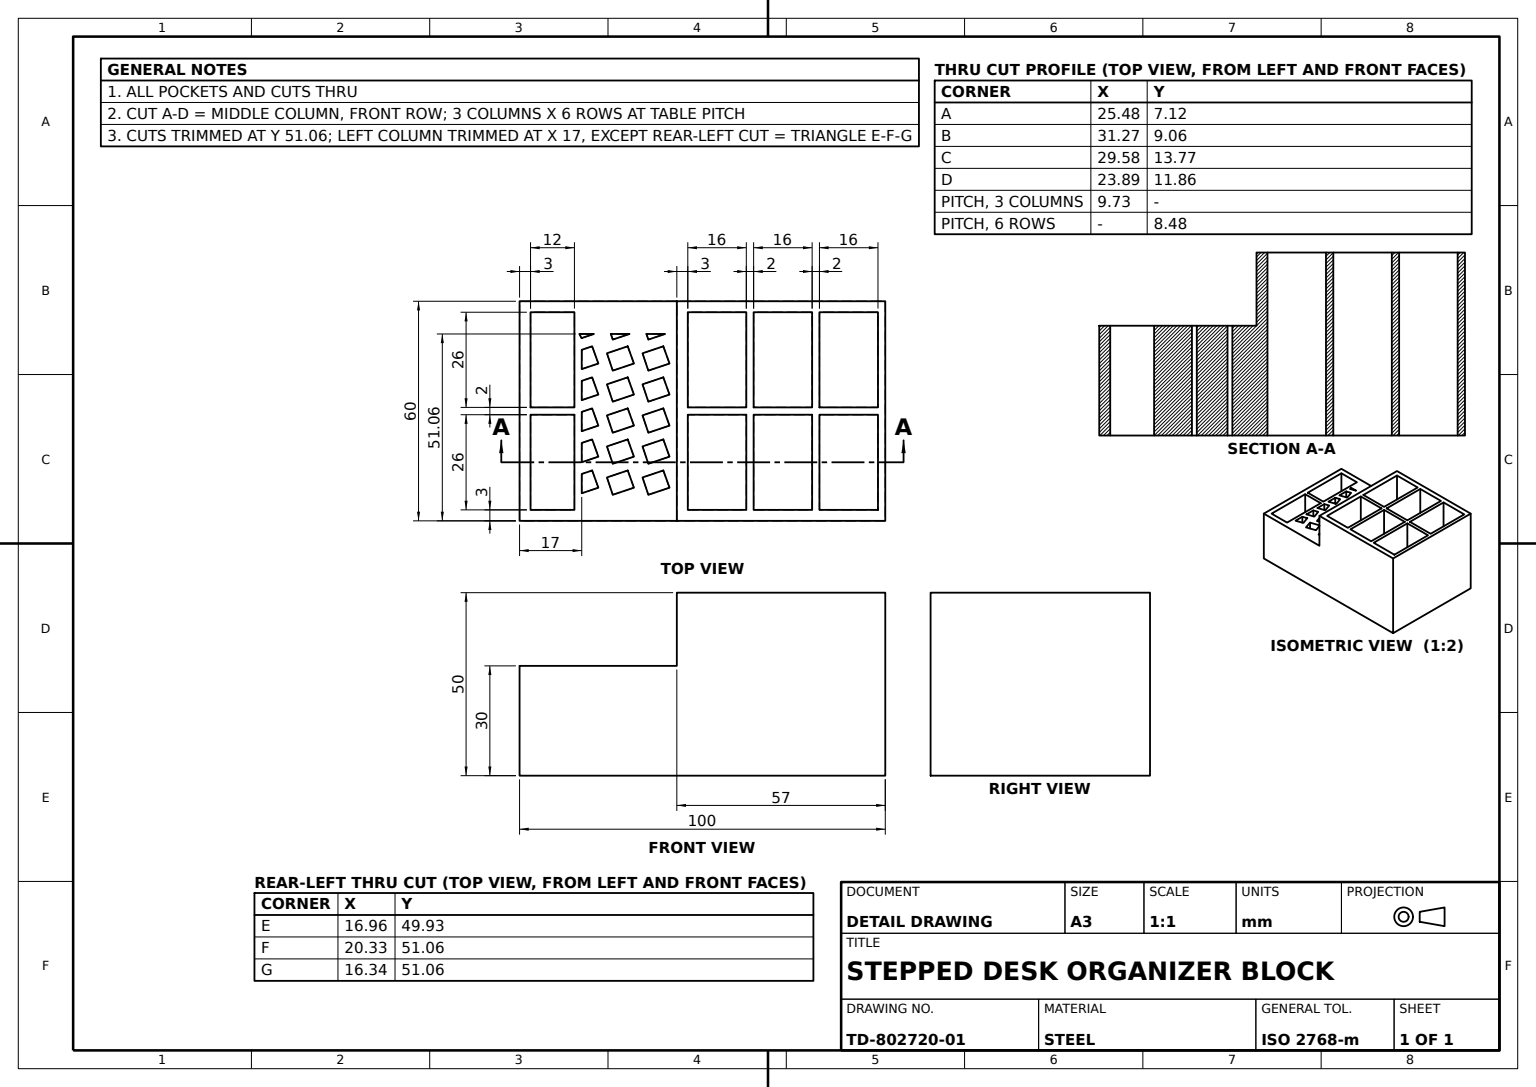
solid
v1 (12,5.599473,-1)
v2 (12,5.599473,-27)
e1 v1 v2 LINE
v3 (12,55.599473,-1)
e2 v1 v3 LINE
v4 (12,55.599473,-27)
e3 v3 v4 LINE
e4 v2 v4 LINE
face PLANE(AX(P(12,5.599473,-1),D(1,0,0),D(0,1,0))) rev [-e1 e2 e3 -e4]
v5 (30,5.599473,-27)
v6 (14,5.599473,-27)
e5 v5 v6 LINE
v7 (30,55.599473,-27)
e6 v5 v7 LINE
v8 (14,55.599473,-27)
e7 v7 v8 LINE
e8 v6 v8 LINE
face PLANE(AX(P(14,5.599473,-27),D(0,0,-1),D(-1,0,0))) rev [-e5 e6 e7 -e8]
v9 (-30.149435,35.599473,-0.727667)
v10 (-33,35.599473,0.227423)
e9 v9 v10 LINE
v11 (-33,5.599473,0.227423)
e10 v11 v10 LINE
v12 (-30.149435,5.599473,-0.727667)
e11 v11 v12 LINE
e12 v12 v9 LINE
face PLANE(AX(P(-33,-4.332499,0.227423),D(-0.317694802,0,-0.948193025),D(-0.948193025,0,0.317694802))) rev [e9 -e10 e11 e12]
v13 (-28.457896,5.599473,3.977511)
e13 v12 v13 LINE
v14 (-28.457896,35.599473,3.977511)
e14 v13 v14 LINE
e15 v14 v9 LINE
face PLANE(AX(P(-30.149435,-4.332499,-0.727667),D(0.941035568,0,-0.338307639),D(-0.338307639,0,-0.941035568))) rev [e13 e14 e15 -e12]
v15 (-4,55.599473,-27)
v16 (-4,55.599473,-1)
e16 v15 v16 LINE
v17 (-4,5.599473,-1)
e17 v17 v16 LINE
v18 (-4,5.599473,-27)
e18 v18 v17 LINE
e19 v18 v15 LINE
face PLANE(AX(P(-4,5.599473,-1),D(-1,0,0),D(0,-1,0))) rev [e16 -e17 -e18 e19]
e20 v4 v15 LINE
e21 v2 v18 LINE
face PLANE(AX(P(-4,5.599473,-27),D(0,0,-1),D(-1,0,0))) rev [e4 e20 -e19 -e21]
v19 (30,5.599473,1)
v20 (30,55.599473,1)
e22 v19 v20 LINE
v21 (14,55.599473,1)
e23 v20 v21 LINE
v22 (14,5.599473,1)
e24 v22 v21 LINE
e25 v19 v22 LINE
face PLANE(AX(P(14,5.599473,1),D(0,0,-1),D(-1,0,0))) rev [e22 e23 -e24 -e25]
v23 (14,55.599473,27)
v24 (30,55.599473,27)
e26 v23 v24 LINE
e27 v21 v23 LINE
e28 v24 v20 LINE
v25 (30,55.599473,-1)
e29 v25 v7 LINE
v26 (14,55.599473,-1)
e30 v26 v25 LINE
e31 v8 v26 LINE
v27 (12,55.599473,27)
v28 (12,55.599473,1)
e32 v27 v28 LINE
v29 (-4,55.599473,27)
e33 v29 v27 LINE
v30 (-4,55.599473,1)
e34 v30 v29 LINE
e35 v28 v30 LINE
v31 (32,55.599473,-1)
v32 (48,55.599473,-1)
e36 v31 v32 LINE
v33 (32,55.599473,-27)
e37 v33 v31 LINE
v34 (48,55.599473,-27)
e38 v34 v33 LINE
e39 v32 v34 LINE
e40 v16 v3 LINE
v35 (48,55.599473,27)
v36 (48,55.599473,1)
e41 v35 v36 LINE
v37 (32,55.599473,27)
e42 v37 v35 LINE
v38 (32,55.599473,1)
e43 v38 v37 LINE
e44 v36 v38 LINE
v39 (50,55.599473,30)
v40 (50,55.599473,-30)
e45 v39 v40 LINE
v41 (-7,55.599473,-30)
e46 v40 v41 LINE
v42 (-7,55.599473,30)
e47 v42 v41 LINE
e48 v39 v42 LINE
face PLANE(AX(P(50,55.599473,30),D(0,-1,0),D(1,0,0))) rev [-e26 -e27 -e23 -e28] [-e29 -e30 -e31 -e7] [-e32 -e33 -e34 -e35] [-e36 -e37 -e38 -e39] [-e20 -e3 -e40 -e16] [-e41 -e42 -e43 -e44] [e45 e46 -e47 -e48]
v43 (-10.691538,35.599473,16.234119)
v44 (-16.380696,35.599473,18.140288)
e49 v43 v44 LINE
v45 (-16.380696,5.599473,18.140288)
e50 v45 v44 LINE
v46 (-10.691538,5.599473,16.234119)
e51 v45 v46 LINE
e52 v46 v43 LINE
face PLANE(AX(P(-16.380696,-4.332499,18.140288),D(-0.317694802,0,-0.948193025),D(-0.948193025,0,0.317694802))) rev [e49 -e50 e51 e52]
v47 (-9,5.599473,-12.984275)
v48 (-9,35.599473,-12.984275)
e53 v47 v48 LINE
v49 (-10.691538,35.599473,-17.689453)
e54 v48 v49 LINE
v50 (-10.691538,5.599473,-17.689453)
e55 v50 v49 LINE
e56 v50 v47 LINE
face PLANE(AX(P(-10.691538,-4.332499,-17.689453),D(0.941035568,0,-0.338307639),D(-0.338307639,0,-0.941035568))) rev [e53 e54 -e55 e56]
v51 (-33,35.599473,-8.25347)
v52 (-33,35.599473,-2.981537)
e57 v51 v52 LINE
v53 (-33,5.599473,-2.981537)
e58 v53 v52 LINE
v54 (-33,5.599473,-8.25347)
e59 v53 v54 LINE
e60 v54 v51 LINE
face PLANE(AX(P(-33,-4.332499,-8.25347),D(-1,0,0),D(0,-1,0))) rev [e57 -e58 e59 e60]
v55 (-24.521549,35.599473,5.918339)
v56 (-18.728948,35.599473,3.977511)
e61 v55 v56 LINE
v57 (-18.728948,5.599473,3.977511)
e62 v57 v56 LINE
v58 (-24.521549,5.599473,5.918339)
e63 v57 v58 LINE
e64 v58 v55 LINE
face PLANE(AX(P(-18.728948,-4.332499,3.977511),D(0.317694802,0,0.948193025),D(0.948193025,0,-0.317694802))) rev [e61 -e62 e63 e64]
v59 (-33.041679,5.599473,-19.929358)
v60 (-33.663374,5.599473,-21.060067)
e65 v59 v60 LINE
v61 (-33.663374,35.599473,-21.060067)
e66 v60 v61 LINE
v62 (-33.041679,35.599473,-19.929358)
e67 v61 v62 LINE
e68 v59 v62 LINE
face PLANE(AX(P(-33.041679,-4.332499,-19.929358),D(-0.87627987,0,0.481802437),D(0.481802437,0,0.87627987))) rev [e65 e66 e67 -e68]
v63 (-10.691538,35.599473,7.753226)
v64 (-16.380696,35.599473,9.659395)
e69 v63 v64 LINE
v65 (-16.380696,5.599473,9.659395)
e70 v65 v64 LINE
v66 (-10.691538,5.599473,7.753226)
e71 v65 v66 LINE
e72 v66 v63 LINE
face PLANE(AX(P(-16.380696,-4.332499,9.659395),D(-0.317694802,0,-0.948193025),D(-0.948193025,0,0.317694802))) rev [e69 -e70 e71 e72]
v67 (32,5.599473,27)
e73 v67 v37 LINE
v68 (32,5.599473,1)
e74 v68 v67 LINE
e75 v68 v38 LINE
face PLANE(AX(P(32,5.599473,1),D(-1,0,0),D(0,-1,0))) rev [-e73 -e74 e75 e43]
v69 (-28.457896,35.599473,-12.984275)
v70 (-30.149435,35.599473,-17.689453)
e76 v69 v70 LINE
v71 (-30.149435,5.599473,-17.689453)
e77 v71 v70 LINE
v72 (-28.457896,5.599473,-12.984275)
e78 v71 v72 LINE
e79 v72 v69 LINE
face PLANE(AX(P(-30.149435,-4.332499,-17.689453),D(0.941035568,0,-0.338307639),D(-0.338307639,0,-0.941035568))) rev [e76 -e77 e78 e79]
v73 (-9,5.599473,3.977511)
v74 (-14.7926,5.599473,5.918339)
e80 v73 v74 LINE
v75 (-14.7926,35.599473,5.918339)
e81 v74 v75 LINE
v76 (-9,35.599473,3.977511)
e82 v75 v76 LINE
e83 v73 v76 LINE
face PLANE(AX(P(-9,-4.332499,3.977511),D(0.317694802,0,0.948193025),D(0.948193025,0,-0.317694802))) rev [e80 e81 e82 -e83]
v77 (-4,5.599473,1)
e84 v77 v30 LINE
v78 (-4,5.599473,27)
e85 v78 v29 LINE
e86 v77 v78 LINE
face PLANE(AX(P(-4,5.599473,1),D(-1,0,0),D(0,-1,0))) rev [e84 e34 -e85 -e86]
e87 v17 v1 LINE
face PLANE(AX(P(-4,5.599473,-1),D(0,0,1),D(1,0,0))) rev [-e2 -e87 e17 e40]
v79 (-24.521549,35.599473,-11.043447)
v80 (-18.728948,35.599473,-12.984275)
e88 v79 v80 LINE
v81 (-18.728948,5.599473,-12.984275)
e89 v81 v80 LINE
v82 (-24.521549,5.599473,-11.043447)
e90 v81 v82 LINE
e91 v82 v79 LINE
face PLANE(AX(P(-18.728948,-4.332499,-12.984275),D(0.317694802,0,0.948193025),D(0.948193025,0,-0.317694802))) rev [e88 -e89 e90 e91]
v83 (-20.420486,5.599473,-9.20856)
v84 (-20.420486,35.599473,-9.20856)
e92 v83 v84 LINE
v85 (-26.109645,35.599473,-7.302391)
e93 v84 v85 LINE
v86 (-26.109645,5.599473,-7.302391)
e94 v86 v85 LINE
e95 v86 v83 LINE
face PLANE(AX(P(-26.109645,-4.332499,-7.302391),D(-0.317694802,0,-0.948193025),D(-0.948193025,0,0.317694802))) rev [e92 e93 -e94 e95]
v87 (48,5.599473,1)
e96 v87 v36 LINE
v88 (48,5.599473,27)
e97 v88 v87 LINE
e98 v88 v35 LINE
face PLANE(AX(P(48,5.599473,1),D(1,0,0),D(0,1,0))) rev [e41 -e96 -e97 e98]
v89 (-33,5.599473,17.189209)
v90 (-33,35.599473,17.189209)
e99 v89 v90 LINE
v91 (-30.149435,5.599473,16.234119)
e100 v89 v91 LINE
v92 (-30.149435,35.599473,16.234119)
e101 v91 v92 LINE
e102 v92 v90 LINE
face PLANE(AX(P(-33,-4.332499,17.189209),D(-0.317694802,0,-0.948193025),D(-0.948193025,0,0.317694802))) rev [-e99 e100 e101 e102]
v93 (-14.7926,35.599473,-2.562554)
v94 (-9,35.599473,-4.503382)
e103 v93 v94 LINE
v95 (-9,5.599473,-4.503382)
e104 v95 v94 LINE
v96 (-14.7926,5.599473,-2.562554)
e105 v95 v96 LINE
e106 v96 v93 LINE
face PLANE(AX(P(-9,-4.332499,-4.503382),D(0.317694802,0,0.948193025),D(0.948193025,0,-0.317694802))) rev [e103 -e104 e105 e106]
v97 (-47,5.599473,-1)
v98 (-35,5.599473,-1)
e107 v97 v98 LINE
v99 (-47,35.599473,-1)
e108 v97 v99 LINE
v100 (-35,35.599473,-1)
e109 v99 v100 LINE
e110 v98 v100 LINE
face PLANE(AX(P(-47,5.599473,-1),D(0,0,1),D(1,0,0))) rev [-e107 e108 e109 -e110]
v101 (-9,5.599473,20.939297)
e111 v46 v101 LINE
v102 (-9,35.599473,20.939297)
e112 v101 v102 LINE
e113 v102 v43 LINE
face PLANE(AX(P(-10.691538,-4.332499,16.234119),D(0.941035568,0,-0.338307639),D(-0.338307639,0,-0.941035568))) rev [e111 e112 e113 -e52]
v103 (-14.7926,35.599473,14.399231)
e114 v64 v103 LINE
v104 (-14.7926,5.599473,14.399231)
e115 v104 v103 LINE
e116 v104 v65 LINE
face PLANE(AX(P(-14.7926,-4.332499,14.399231),D(-0.948193025,0,0.317694802),D(0.317694802,0,0.948193025))) rev [e114 -e115 e116 e70]
v105 (-47,5.599473,27)
v106 (-47,35.599473,27)
e117 v105 v106 LINE
v107 (-47,5.599473,1)
e118 v107 v105 LINE
v108 (-47,35.599473,1)
e119 v107 v108 LINE
e120 v108 v106 LINE
face PLANE(AX(P(-47,5.599473,27),D(-1,0,0),D(0,-1,0))) rev [-e117 -e118 e119 e120]
v109 (-24.521549,5.599473,14.399231)
v110 (-24.521549,35.599473,14.399231)
e121 v109 v110 LINE
v111 (-26.109645,5.599473,9.659395)
e122 v109 v111 LINE
v112 (-26.109645,35.599473,9.659395)
e123 v111 v112 LINE
e124 v112 v110 LINE
face PLANE(AX(P(-24.521549,-4.332499,14.399231),D(-0.948193025,0,0.317694802),D(0.317694802,0,0.948193025))) rev [-e121 e122 e123 e124]
v113 (-14.7926,5.599473,-11.043447)
e125 v47 v113 LINE
v114 (-14.7926,35.599473,-11.043447)
e126 v113 v114 LINE
e127 v114 v48 LINE
face PLANE(AX(P(-9,-4.332499,-12.984275),D(0.317694802,0,0.948193025),D(0.948193025,0,-0.317694802))) rev [e125 e126 e127 -e53]
v115 (14,5.599473,27)
e128 v115 v23 LINE
e129 v22 v115 LINE
face PLANE(AX(P(14,5.599473,1),D(-1,0,0),D(0,-1,0))) rev [e24 e27 -e128 -e129]
v116 (-24.521549,35.599473,-19.52434)
v117 (-19.938013,35.599473,-21.060067)
e130 v116 v117 LINE
v118 (-19.938013,5.599473,-21.060067)
e131 v118 v117 LINE
v119 (-24.521549,5.599473,-19.52434)
e132 v118 v119 LINE
e133 v119 v116 LINE
face PLANE(AX(P(-19.938013,-4.332499,-21.060067),D(0.317694802,0,0.948193025),D(0.948193025,0,-0.317694802))) rev [e130 -e131 e132 e133]
v120 (-28.457896,35.599473,-4.503382)
e134 v52 v120 LINE
v121 (-28.457896,5.599473,-4.503382)
e135 v121 v120 LINE
e136 v121 v53 LINE
face PLANE(AX(P(-28.457896,-4.332499,-4.503382),D(0.317694802,0,0.948193025),D(0.948193025,0,-0.317694802))) rev [e58 e134 -e135 e136]
v122 (-33,35.599473,22.461142)
e137 v90 v122 LINE
v123 (-33,5.599473,22.461142)
e138 v123 v122 LINE
e139 v123 v89 LINE
face PLANE(AX(P(-33,-4.332499,17.189209),D(-1,0,0),D(0,-1,0))) rev [e99 e137 -e138 e139]
v124 (-28.457896,5.599473,20.939297)
v125 (-28.457896,35.599473,20.939297)
e140 v124 v125 LINE
e141 v125 v92 LINE
e142 v91 v124 LINE
face PLANE(AX(P(-30.149435,-4.332499,16.234119),D(0.941035568,0,-0.338307639),D(-0.338307639,0,-0.941035568))) rev [e140 e141 -e101 e142]
v126 (-16.380696,5.599473,1.178502)
v127 (-10.691538,5.599473,-0.727667)
e143 v126 v127 LINE
v128 (-10.691538,35.599473,-0.727667)
e144 v127 v128 LINE
v129 (-16.380696,35.599473,1.178502)
e145 v128 v129 LINE
e146 v126 v129 LINE
face PLANE(AX(P(-16.380696,-4.332499,1.178502),D(-0.317694802,0,-0.948193025),D(-0.948193025,0,0.317694802))) rev [e143 e144 e145 -e146]
v130 (-29.666962,5.599473,-21.060067)
e147 v60 v130 LINE
v131 (-29.666962,35.599473,-21.060067)
e148 v130 v131 LINE
e149 v131 v61 LINE
face PLANE(AX(P(-33.663374,-4.332499,-21.060067),D(0,0,-1),D(-1,0,0))) rev [-e66 e147 e148 e149]
v132 (-30.149435,5.599473,7.753226)
v133 (-28.457896,5.599473,12.458404)
e150 v132 v133 LINE
v134 (-28.457896,35.599473,12.458404)
e151 v133 v134 LINE
v135 (-30.149435,35.599473,7.753226)
e152 v134 v135 LINE
e153 v132 v135 LINE
face PLANE(AX(P(-30.149435,-4.332499,7.753226),D(0.941035568,0,-0.338307639),D(-0.338307639,0,-0.941035568))) rev [e150 e151 e152 -e153]
v136 (-7,35.599473,30)
e154 v42 v136 LINE
v137 (-50,35.599473,30)
e155 v136 v137 LINE
v138 (-50,5.599473,30)
e156 v137 v138 LINE
v139 (50,5.599473,30)
e157 v138 v139 LINE
e158 v139 v39 LINE
face PLANE(AX(P(0,0,30),D(0,0,1),D(1,0,0))) [e48 e154 e155 e156 e157 e158]
v140 (-33,5.599473,13.980249)
e159 v133 v140 LINE
v141 (-33,35.599473,13.980249)
e160 v140 v141 LINE
e161 v141 v134 LINE
face PLANE(AX(P(-28.457896,-4.332499,12.458404),D(0.317694802,0,0.948193025),D(0.948193025,0,-0.317694802))) rev [-e151 e159 e160 e161]
v142 (30,5.599473,-1)
e162 v142 v5 LINE
e163 v142 v25 LINE
face PLANE(AX(P(30,5.599473,-1),D(1,0,0),D(0,1,0))) rev [-e6 -e162 e163 e29]
v143 (-35,35.599473,-27)
v144 (-47,35.599473,-27)
e164 v143 v144 LINE
v145 (-47,5.599473,-27)
e165 v145 v144 LINE
v146 (-35,5.599473,-27)
e166 v146 v145 LINE
e167 v146 v143 LINE
face PLANE(AX(P(-47,5.599473,-27),D(0,0,-1),D(-1,0,0))) rev [e164 -e165 -e166 e167]
v147 (-26.109645,35.599473,-15.783284)
e168 v147 v79 LINE
v148 (-26.109645,5.599473,-15.783284)
e169 v82 v148 LINE
e170 v148 v147 LINE
face PLANE(AX(P(-24.521549,-4.332499,-11.043447),D(-0.948193025,0,0.317694802),D(0.317694802,0,0.948193025))) rev [e168 -e91 e169 e170]
v149 (-33,35.599473,5.499356)
e171 v10 v149 LINE
v150 (-33,5.599473,5.499356)
e172 v150 v149 LINE
e173 v150 v11 LINE
face PLANE(AX(P(-33,-4.332499,0.227423),D(-1,0,0),D(0,-1,0))) rev [e171 -e172 e173 e10]
v151 (-14.7926,5.599473,-19.52434)
v152 (-14.7926,35.599473,-19.52434)
e174 v151 v152 LINE
v153 (-15.30715,5.599473,-21.060067)
e175 v151 v153 LINE
v154 (-15.30715,35.599473,-21.060067)
e176 v153 v154 LINE
e177 v154 v152 LINE
face PLANE(AX(P(-14.7926,-4.332499,-19.52434),D(-0.948193025,0,0.317694802),D(0.317694802,0,0.948193025))) rev [-e174 e175 e176 e177]
e178 v130 v59 LINE
e179 v62 v131 LINE
face PLANE(AX(P(-29.666962,-4.332499,-21.060067),D(0.317694802,0,0.948193025),D(0.948193025,0,-0.317694802))) rev [-e148 e178 e68 e179]
v155 (-24.521549,5.599473,22.880124)
v156 (-24.521549,35.599473,22.880124)
e180 v155 v156 LINE
v157 (-26.109645,5.599473,18.140288)
e181 v155 v157 LINE
v158 (-26.109645,35.599473,18.140288)
e182 v157 v158 LINE
e183 v158 v156 LINE
face PLANE(AX(P(-24.521549,-4.332499,22.880124),D(-0.948193025,0,0.317694802),D(0.317694802,0,0.948193025))) rev [-e180 e181 e182 e183]
e184 v67 v88 LINE
face PLANE(AX(P(32,5.599473,27),D(0,0,1),D(1,0,0))) rev [-e98 -e184 e73 e42]
v159 (48,5.599473,-1)
e185 v159 v32 LINE
v160 (32,5.599473,-1)
e186 v160 v159 LINE
e187 v160 v31 LINE
face PLANE(AX(P(32,5.599473,-1),D(0,0,1),D(1,0,0))) rev [e36 -e185 -e186 e187]
v161 (-16.380696,5.599473,-7.302391)
v162 (-16.380696,35.599473,-7.302391)
e188 v161 v162 LINE
e189 v162 v93 LINE
e190 v96 v161 LINE
face PLANE(AX(P(-14.7926,-4.332499,-2.562554),D(-0.948193025,0,0.317694802),D(0.317694802,0,0.948193025))) rev [e188 e189 -e106 e190]
v163 (48,5.599473,-27)
e191 v163 v34 LINE
e192 v159 v163 LINE
face PLANE(AX(P(48,5.599473,-1),D(1,0,0),D(0,1,0))) rev [e39 -e191 -e192 e185]
v164 (12,5.599473,27)
e193 v164 v27 LINE
e194 v78 v164 LINE
face PLANE(AX(P(-4,5.599473,27),D(0,0,1),D(1,0,0))) rev [e33 -e193 -e194 e85]
v165 (-10.691538,35.599473,-9.20856)
e195 v165 v162 LINE
v166 (-10.691538,5.599473,-9.20856)
e196 v161 v166 LINE
e197 v166 v165 LINE
face PLANE(AX(P(-16.380696,-4.332499,-7.302391),D(-0.317694802,0,-0.948193025),D(-0.948193025,0,0.317694802))) rev [e195 -e188 e196 e197]
e198 v124 v123 LINE
e199 v122 v125 LINE
face PLANE(AX(P(-28.457896,-4.332499,20.939297),D(0.317694802,0,0.948193025),D(0.948193025,0,-0.317694802))) rev [-e140 e198 e138 e199]
e200 v100 v143 LINE
e201 v98 v146 LINE
face PLANE(AX(P(-35,5.599473,-27),D(1,0,0),D(0,1,0))) rev [e200 -e167 -e201 e110]
v167 (-18.728948,35.599473,12.458404)
v168 (-20.420486,35.599473,7.753226)
e202 v167 v168 LINE
v169 (-20.420486,5.599473,7.753226)
e203 v169 v168 LINE
v170 (-18.728948,5.599473,12.458404)
e204 v169 v170 LINE
e205 v170 v167 LINE
face PLANE(AX(P(-20.420486,-4.332499,7.753226),D(0.941035568,0,-0.338307639),D(-0.338307639,0,-0.941035568))) rev [e202 -e203 e204 e205]
v171 (-25.036098,5.599473,-21.060067)
e206 v171 v118 LINE
v172 (-25.036098,35.599473,-21.060067)
e207 v117 v172 LINE
e208 v171 v172 LINE
face PLANE(AX(P(-25.036098,-4.332499,-21.060067),D(0,0,-1),D(-1,0,0))) rev [e206 e131 e207 -e208]
v173 (-26.109645,35.599473,1.178502)
e209 v173 v55 LINE
v174 (-26.109645,5.599473,1.178502)
e210 v58 v174 LINE
e211 v174 v173 LINE
face PLANE(AX(P(-24.521549,-4.332499,5.918339),D(-0.948193025,0,0.317694802),D(0.317694802,0,0.948193025))) rev [e209 -e64 e210 e211]
v175 (-14.7926,35.599473,22.880124)
e212 v44 v175 LINE
v176 (-14.7926,5.599473,22.880124)
e213 v176 v175 LINE
e214 v176 v45 LINE
face PLANE(AX(P(-14.7926,-4.332499,22.880124),D(-0.948193025,0,0.317694802),D(0.317694802,0,0.948193025))) rev [e50 e212 -e213 e214]
e215 v149 v14 LINE
e216 v13 v150 LINE
face PLANE(AX(P(-28.457896,-4.332499,3.977511),D(0.317694802,0,0.948193025),D(0.948193025,0,-0.317694802))) rev [e215 -e14 e216 e172]
v177 (-20.420486,5.599473,-17.689453)
v178 (-20.420486,35.599473,-17.689453)
e217 v177 v178 LINE
e218 v177 v81 LINE
e219 v80 v178 LINE
face PLANE(AX(P(-20.420486,-4.332499,-17.689453),D(0.941035568,0,-0.338307639),D(-0.338307639,0,-0.941035568))) rev [-e217 e218 e89 e219]
v179 (-33,5.599473,-11.46243)
e220 v72 v179 LINE
v180 (-33,35.599473,-11.46243)
e221 v179 v180 LINE
e222 v180 v69 LINE
face PLANE(AX(P(-28.457896,-4.332499,-12.984275),D(0.317694802,0,0.948193025),D(0.948193025,0,-0.317694802))) rev [-e79 e220 e221 e222]
e223 v111 v169 LINE
e224 v168 v112 LINE
face PLANE(AX(P(-26.109645,-4.332499,9.659395),D(-0.317694802,0,-0.948193025),D(-0.948193025,0,0.317694802))) rev [e223 e203 e224 -e123]
v181 (50,5.599473,-30)
e225 v181 v40 LINE
e226 v139 v181 LINE
face PLANE(AX(P(50,5.599473,30),D(-1,0,0),D(0,0,1))) rev [e225 -e45 -e158 e226]
v182 (-33,35.599473,-16.734362)
e227 v70 v182 LINE
v183 (-33,5.599473,-16.734362)
e228 v183 v182 LINE
e229 v183 v71 LINE
face PLANE(AX(P(-33,-4.332499,-16.734362),D(-0.317694802,0,-0.948193025),D(-0.948193025,0,0.317694802))) rev [e227 -e228 e229 e77]
v184 (-35,5.599473,27)
v185 (-35,35.599473,27)
e230 v184 v185 LINE
v186 (-35,35.599473,1)
e231 v185 v186 LINE
v187 (-35,5.599473,1)
e232 v187 v186 LINE
e233 v184 v187 LINE
face PLANE(AX(P(-35,5.599473,27),D(1,0,0),D(0,1,0))) rev [e230 e231 -e232 -e233]
v188 (30,5.599473,27)
e234 v188 v19 LINE
e235 v188 v24 LINE
face PLANE(AX(P(30,5.599473,1),D(1,0,0),D(0,1,0))) rev [e28 -e22 -e234 e235]
v189 (-18.728948,35.599473,20.939297)
e236 v156 v189 LINE
v190 (-18.728948,5.599473,20.939297)
e237 v190 v189 LINE
e238 v190 v155 LINE
face PLANE(AX(P(-18.728948,-4.332499,20.939297),D(0.317694802,0,0.948193025),D(0.948193025,0,-0.317694802))) rev [e180 e236 -e237 e238]
v191 (-50,5.599473,-30)
e239 v191 v181 LINE
v192 (-50,35.599473,-30)
e240 v192 v191 LINE
v193 (-7,35.599473,-30)
e241 v193 v192 LINE
e242 v41 v193 LINE
face PLANE(AX(P(0,0,-30),D(0,0,1),D(1,0,0))) rev [-e46 -e225 -e239 -e240 -e241 -e242]
v194 (-16.380696,5.599473,-15.783284)
e243 v194 v50 LINE
e244 v113 v194 LINE
v195 (32,5.599473,-27)
e245 v163 v195 LINE
e246 v195 v160 LINE
e247 v170 v109 LINE
e248 v119 v171 LINE
e249 v87 v68 LINE
v196 (-9,5.599473,12.458404)
e250 v196 v104 LINE
e251 v66 v196 LINE
v197 (-33,5.599473,8.708316)
e252 v197 v132 LINE
e253 v140 v197 LINE
e254 v166 v95 LINE
v198 (-20.420486,5.599473,16.234119)
e255 v198 v190 LINE
e256 v157 v198 LINE
e257 v148 v177 LINE
v199 (-20.420486,5.599473,-0.727667)
e258 v199 v57 LINE
e259 v174 v199 LINE
v200 (12,5.599473,1)
e260 v164 v200 LINE
e261 v200 v77 LINE
e262 v138 v191 LINE
v201 (14,5.599473,-1)
e263 v6 v201 LINE
e264 v201 v142 LINE
e265 v145 v97 LINE
e266 v101 v176 LINE
v202 (-24.521549,5.599473,-2.562554)
e267 v202 v86 LINE
v203 (-18.728948,5.599473,-4.503382)
e268 v203 v202 LINE
e269 v83 v203 LINE
e270 v74 v126 LINE
e271 v127 v73 LINE
e272 v187 v107 LINE
e273 v105 v184 LINE
v204 (-10.209065,5.599473,-21.060067)
e274 v204 v151 LINE
e275 v153 v204 LINE
v205 (-30.149435,5.599473,-9.20856)
e276 v205 v121 LINE
e277 v54 v205 LINE
e278 v179 v183 LINE
e279 v115 v188 LINE
face PLANE(AX(P(-50,5.599473,30),D(0,1,0),D(-1,0,0))) rev [-e147 -e65 -e178] [-e13 -e11 -e173 -e216] [-e243 -e244 -e125 -e56] [e192 e245 e246 e186] [-e122 -e247 -e204 -e223] [-e248 -e132 -e206] [e74 e184 e97 e249] [-e116 -e250 -e251 -e71] [-e252 -e253 -e159 -e150] [-e254 -e196 -e190 -e105] [-e255 -e256 -e181 -e238] [-e100 -e139 -e198 -e142] [-e257 -e169 -e90 -e218] [-e63 -e258 -e259 -e210] [e260 e261 e86 e194] [e262 e239 -e226 -e157] [e162 e5 e263 e264] [e201 e166 e265 e107] [-e51 -e214 -e266 -e111] [-e95 -e267 -e268 -e269] [-e143 -e270 -e80 -e271] [e233 e272 e118 e273] [-e175 -e274 -e275] [-e276 -e277 -e59 -e136] [-e278 -e220 -e78 -e229] [e25 e129 e279 e234] [e18 e87 e1 e21]
e280 v129 v75 LINE
face PLANE(AX(P(-14.7926,-4.332499,5.918339),D(-0.948193025,0,0.317694802),D(0.317694802,0,0.948193025))) rev [-e81 e270 e146 e280]
e281 v201 v26 LINE
face PLANE(AX(P(14,5.599473,-1),D(-1,0,0),D(0,-1,0))) rev [e8 e31 -e281 -e263]
v206 (-20.420486,35.599473,16.234119)
e282 v189 v206 LINE
e283 v198 v206 LINE
face PLANE(AX(P(-20.420486,-4.332499,16.234119),D(0.941035568,0,-0.338307639),D(-0.338307639,0,-0.941035568))) rev [e255 e237 e282 -e283]
v207 (-16.380696,35.599473,-15.783284)
e284 v194 v207 LINE
e285 v207 v114 LINE
face PLANE(AX(P(-14.7926,-4.332499,-11.043447),D(-0.948193025,0,0.317694802),D(0.317694802,0,0.948193025))) rev [e284 e285 -e126 e244]
e286 v186 v108 LINE
face PLANE(AX(P(-47,5.599473,1),D(0,0,-1),D(-1,0,0))) rev [-e272 e232 e286 -e119]
face PLANE(AX(P(32,5.599473,1),D(0,0,-1),D(-1,0,0))) rev [e44 -e75 -e249 e96]
e287 v106 v185 LINE
face PLANE(AX(P(-47,5.599473,27),D(0,0,1),D(1,0,0))) rev [e117 e287 -e230 -e273]
v208 (-10.209065,35.599473,-21.060067)
e288 v204 v208 LINE
e289 v152 v208 LINE
face PLANE(AX(P(-10.209065,-4.332499,-21.060067),D(0.317694802,0,0.948193025),D(0.948193025,0,-0.317694802))) rev [-e288 e274 e174 e289]
e290 v206 v158 LINE
face PLANE(AX(P(-26.109645,-4.332499,18.140288),D(-0.317694802,0,-0.948193025),D(-0.948193025,0,0.317694802))) rev [-e182 e256 e283 e290]
e291 v76 v128 LINE
face PLANE(AX(P(-10.691538,-4.332499,-0.727667),D(0.941035568,0,-0.338307639),D(-0.338307639,0,-0.941035568))) rev [-e144 e271 e83 e291]
e292 v49 v207 LINE
face PLANE(AX(P(-16.380696,-4.332499,-15.783284),D(-0.317694802,0,-0.948193025),D(-0.948193025,0,0.317694802))) rev [e243 e55 e292 -e284]
e293 v110 v167 LINE
face PLANE(AX(P(-18.728948,-4.332499,12.458404),D(0.317694802,0,0.948193025),D(0.948193025,0,-0.317694802))) rev [-e205 e247 e121 e293]
e294 v200 v28 LINE
face PLANE(AX(P(-4,5.599473,1),D(0,0,-1),D(-1,0,0))) rev [e35 -e84 -e261 e294]
e295 v144 v99 LINE
face PLANE(AX(P(-47,5.599473,-27),D(-1,0,0),D(0,-1,0))) rev [-e265 e165 e295 -e108]
e296 v172 v116 LINE
face PLANE(AX(P(-24.521549,-4.332499,-19.52434),D(-0.948193025,0,0.317694802),D(0.317694802,0,0.948193025))) rev [-e133 e248 e208 e296]
v209 (-24.521549,35.599473,-2.562554)
e297 v85 v209 LINE
e298 v202 v209 LINE
face PLANE(AX(P(-24.521549,-4.332499,-2.562554),D(-0.948193025,0,0.317694802),D(0.317694802,0,0.948193025))) rev [e94 e297 -e298 e267]
e299 v136 v193 LINE
face PLANE(AX(P(-7,55.599473,30),D(1,0,0),D(0,0,-1))) rev [e242 -e299 -e154 e47]
v210 (-33,35.599473,8.708316)
e300 v135 v210 LINE
e301 v197 v210 LINE
face PLANE(AX(P(-33,-4.332499,8.708316),D(-0.317694802,0,-0.948193025),D(-0.948193025,0,0.317694802))) rev [e153 e300 -e301 e252]
e302 v182 v180 LINE
face PLANE(AX(P(-33,-4.332499,-16.734362),D(-1,0,0),D(0,-1,0))) rev [-e221 e278 e228 e302]
v211 (-20.420486,35.599473,-0.727667)
e303 v199 v211 LINE
e304 v211 v173 LINE
face PLANE(AX(P(-26.109645,-4.332499,1.178502),D(-0.317694802,0,-0.948193025),D(-0.948193025,0,0.317694802))) rev [e259 e303 e304 -e211]
face PLANE(AX(P(14,5.599473,27),D(0,0,1),D(1,0,0))) rev [e26 -e235 -e279 e128]
e305 v208 v154 LINE
face PLANE(AX(P(-15.30715,-4.332499,-21.060067),D(0,0,-1),D(-1,0,0))) rev [-e176 e275 e288 e305]
e306 v137 v192 LINE
face PLANE(AX(P(-50,35.599473,30),D(1,0,0),D(0,1,0))) rev [-e156 e306 e240 -e262]
e307 v56 v211 LINE
face PLANE(AX(P(-20.420486,-4.332499,-0.727667),D(0.941035568,0,-0.338307639),D(-0.338307639,0,-0.941035568))) rev [e307 -e303 e258 e62]
v212 (-18.728948,35.599473,-4.503382)
e308 v209 v212 LINE
e309 v203 v212 LINE
face PLANE(AX(P(-18.728948,-4.332499,-4.503382),D(0.317694802,0,0.948193025),D(0.948193025,0,-0.317694802))) rev [e268 e298 e308 -e309]
v213 (-9,35.599473,12.458404)
e310 v196 v213 LINE
e311 v213 v63 LINE
face PLANE(AX(P(-10.691538,-4.332499,7.753226),D(0.941035568,0,-0.338307639),D(-0.338307639,0,-0.941035568))) rev [e251 e310 e311 -e72]
e312 v195 v33 LINE
face PLANE(AX(P(32,5.599473,-1),D(-1,0,0),D(0,-1,0))) rev [-e187 -e246 e312 e37]
e313 v94 v165 LINE
face PLANE(AX(P(-10.691538,-4.332499,-9.20856),D(0.941035568,0,-0.338307639),D(-0.338307639,0,-0.941035568))) rev [e313 -e197 e254 e104]
e314 v210 v141 LINE
face PLANE(AX(P(-33,-4.332499,8.708316),D(-1,0,0),D(0,0,1))) rev [e314 -e160 e253 e301]
e315 v178 v147 LINE
face PLANE(AX(P(-26.109645,-4.332499,-15.783284),D(-0.317694802,0,-0.948193025),D(-0.948193025,0,0.317694802))) rev [-e170 e257 e217 e315]
face PLANE(AX(P(14,5.599473,-1),D(0,0,1),D(1,0,0))) rev [e281 e30 -e163 -e264]
e316 v103 v213 LINE
face PLANE(AX(P(-9,-4.332499,12.458404),D(0.317694802,0,0.948193025),D(0.948193025,0,-0.317694802))) rev [e316 -e310 e250 e115]
v214 (-30.149435,35.599473,-9.20856)
e317 v205 v214 LINE
e318 v214 v51 LINE
face PLANE(AX(P(-33,-4.332499,-8.25347),D(-0.317694802,0,-0.948193025),D(-0.948193025,0,0.317694802))) rev [e317 e318 -e60 e277]
e319 v120 v214 LINE
face PLANE(AX(P(-30.149435,-4.332499,-9.20856),D(0.941035568,0,-0.338307639),D(-0.338307639,0,-0.941035568))) rev [e276 e135 e319 -e317]
face PLANE(AX(P(32,5.599473,-27),D(0,0,-1),D(-1,0,0))) rev [e191 e38 -e312 -e245]
face PLANE(AX(P(12,5.599473,1),D(1,0,0),D(0,1,0))) rev [-e294 -e260 e193 e32]
e320 v175 v102 LINE
e321 v212 v84 LINE
face PLANE(AX(P(-7,35.599473,30),D(0,-1,0),D(1,0,0))) rev [-e113 -e320 -e212 -e49] [-e134 -e57 -e318 -e319] [-e302 -e227 -e76 -e222] [-e179 -e67 -e149] [-e183 -e290 -e282 -e236] [-e93 -e321 -e308 -e297] [-e152 -e161 -e314 -e300] [-e306 -e155 e299 e241] [-e296 -e207 -e130] [-e295 -e164 -e200 -e109] [-e189 -e195 -e313 -e103] [-e202 -e293 -e124 -e224] [-e127 -e285 -e292 -e54] [-e287 -e120 -e286 -e231] [-e177 -e305 -e289] [-e88 -e168 -e315 -e219] [-e102 -e141 -e199 -e137] [-e215 -e171 -e9 -e15] [-e280 -e145 -e291 -e82] [-e209 -e304 -e307 -e61] [-e114 -e69 -e311 -e316]
face PLANE(AX(P(-9,-4.332499,20.939297),D(0.317694802,0,0.948193025),D(0.948193025,0,-0.317694802))) rev [-e112 e266 e213 e320]
face PLANE(AX(P(-20.420486,-4.332499,-9.20856),D(0.941035568,0,-0.338307639),D(-0.338307639,0,-0.941035568))) rev [e321 -e92 e269 e309]
